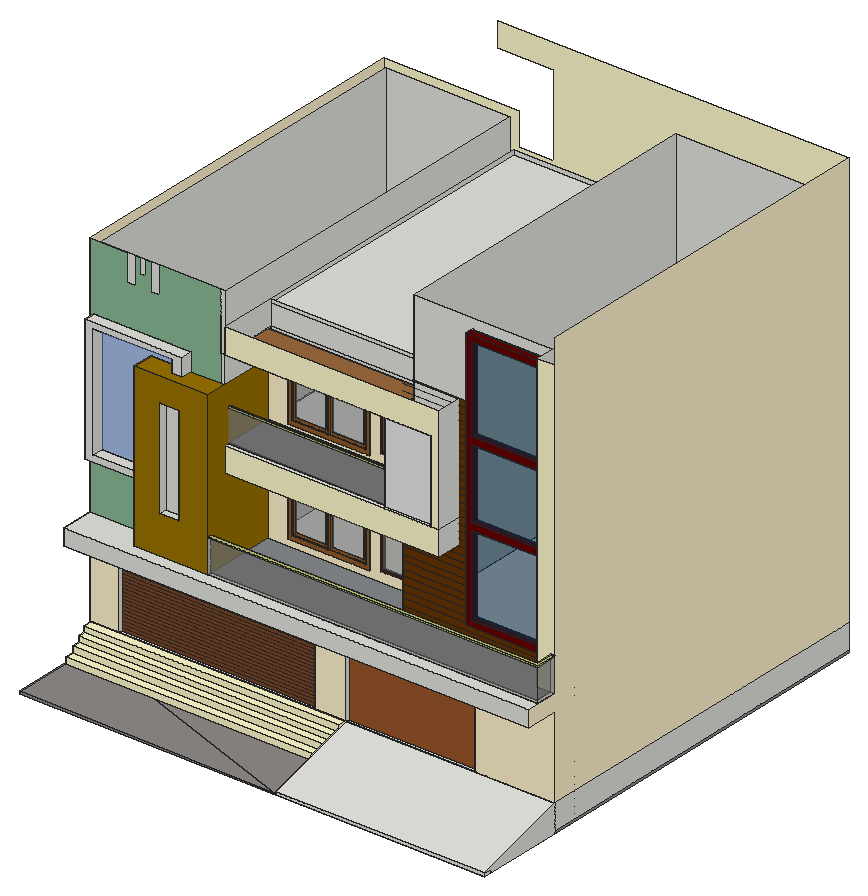
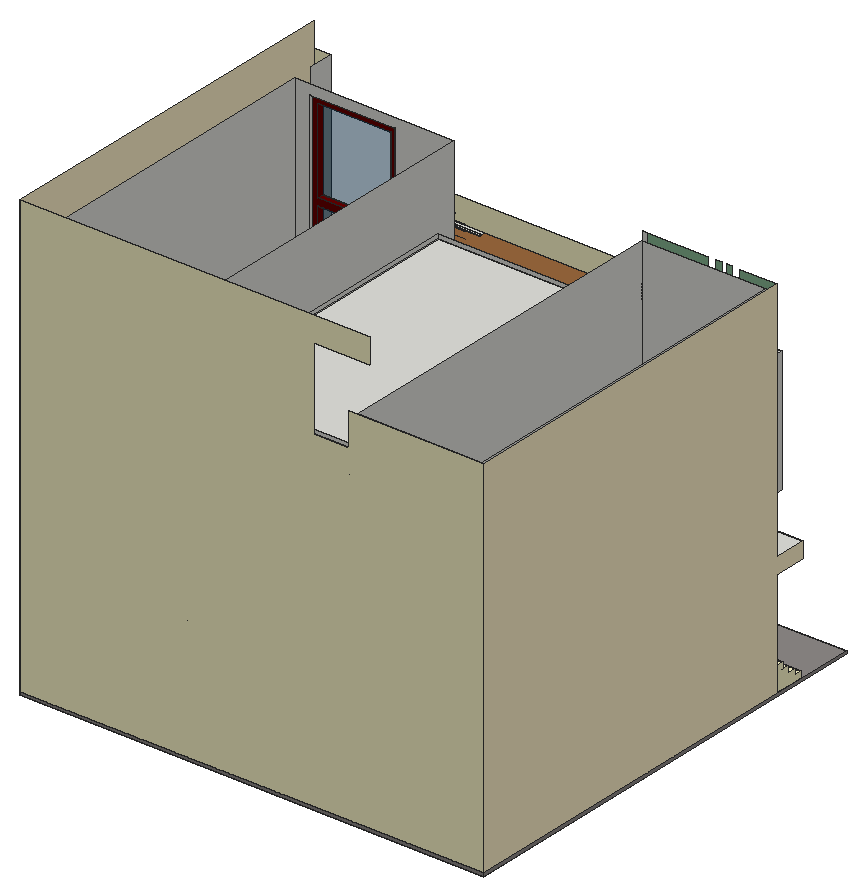
# SketchUp Ruby script. Lengths in inches.
U = 1.inch
M = Sketchup.active_model
def pt(a) = Geom::Point3d.new(a.map { |v| v * U })
def face(e, loops, mat)
  f = e.add_face(loops[0].map { |a| pt(a) })
  loops[1..].each { |l| e.add_face(l.map { |a| pt(a) }).erase! }
  f.material = f.back_material = mat if mat
  f
end
# faces: each face lists its corners as indices into pts; further lists are holes
def faces(e, pts, list, mat = nil) = list.each { |f| face(e, (f[0].is_a?(Array) ? f : [f]).map { |l| l.map { |i| pts[i] } }, mat) }
# xy, xz, yz: faces in a plane at the given z, y or x. An outline is a flat list of corners, or four numbers for a rectangle; further outlines are holes
def ring(l) = l.size == 4 ? [[l[0], l[1]], [l[2], l[1]], [l[2], l[3]], [l[0], l[3]]] : l.each_slice(2).to_a
def flat(e, list, mat, &to3) = list.each { |f| face(e, (f[0].is_a?(Array) ? f : [f]).map { |l| ring(l).map { |u, v| to3.(u, v) } }, mat) }
def xy(e, z, list, mat = nil) = flat(e, list, mat) { |x, y| [x, y, z] }
def xz(e, y, list, mat = nil) = flat(e, list, mat) { |x, z| [x, y, z] }
def yz(e, x, list, mat = nil) = flat(e, list, mat) { |y, z| [x, y, z] }
def lines(e, pts, list) = list.each { |a, b| e.add_line(pt(pts[a]), pt(pts[b])) }
# prism: a flat outline (further loops are holes) pulled along v
def prism(e, loops, v, mat = nil)
  f = face(e, loops, mat); d = Geom::Vector3d.new(v.map { |x| x * U })
  f.pushpull(f.normal.samedirection?(d) ? d.length : -d.length)
end
def box(e, o, s, mat = nil) = prism(e, [[o, [o[0] + s[0], o[1], o[2]], [o[0] + s[0], o[1] + s[1], o[2]], [o[0], o[1] + s[1], o[2]]]], [0, 0, s[2]], mat)
def at(x, y, z, deg = 0) = Geom::Transformation.translation(pt([x, y, z])) * Geom::Transformation.rotation(ORIGIN, Z_AXIS, deg.degrees)
def axes(o, x, y, z) = Geom::Transformation.new([*x, 0, *y, 0, *z, 0, *pt(o).to_a, 1])
def part(name) = M.definitions.add(name)
# library, detail: a bought-in or finely detailed component or shape, given as its bounding box
def library(name, o, s) = part(name).tap { |d| box(d.entities, o, s) }
def detail(e, o, s) = box(e.add_group.entities, o, s)
def put(e, d, t, mat = nil) = e.add_instance(d, t).tap { |i| i.material = mat if mat }
def group(e, t, mat = nil) = e.add_group.tap { |g| g.transformation = t; g.material = mat if mat }.entities
root = M.entities
M.materials.add("[0050_LemonChiffon]").color = [255, 250, 205]
M.materials.add("[0079_Teal]").color = [136, 184, 147]
M.materials.add("[Blacktop Old 01]").color = [132, 136, 139]
M.materials.add("[Color A08]").color = [102, 0, 0]
M.materials.add("[Color B08]").color = [102, 25, 0]
M.materials.add("[Color C08]").color = [102, 51, 0]
M.materials.add("[Color D01]").color = [255, 242, 204]
M.materials.add("[Color D07]").color = [153, 114, 0]
M.materials.add("[Herringbone 2x1]").color = [231, 231, 231]
M.materials.add("[Metal Corrugated Shiny]").color = [193, 193, 113]
M.materials.add("[Stone Marble]").color = [143, 138, 136]
M.materials.add("[Translucent Glass Blue]").color = [4, 53, 86]
M.materials["[Translucent Glass Blue]"].alpha = 0.5
M.materials.add("[Translucent Glass Blue]1").color = [100, 149, 237]
M.materials["[Translucent Glass Blue]1"].alpha = 0.5
M.materials.add("[Translucent Glass Gray]").color = [128, 128, 128]
M.materials["[Translucent Glass Gray]"].alpha = 0.5
M.materials.add("[Wood Cherry Original]").color = [152, 86, 42]
M.materials.add("[Wood Floor Parquet]").color = [145, 89, 39]
M.materials.add("[Wood Floor]").color = [155, 105, 61]
M.materials.add("[Wood Veneer 01]").color = [120, 70, 37]
c1 = part("Group\#2")
xy(c1.entities,0,[[0,0,217.625,6.75],[0,6.75,217.625,8.875]],"[Wood Floor Parquet]")
xy(c1.entities,10.46,[[10.46,0,106.8125,6.75],[108.8125,0,207.17,6.75],[10.46,6.75,106.8125,8.875],[108.8125,6.75,207.17,8.875]],"[Wood Floor Parquet]")
xy(c1.entities,17.65,[[17.65,6.75,99.62,8.875],[116.01,6.75,199.97,8.875]],"[Wood Floor Parquet]")
xy(c1.entities,173.85,[[17.65,6.75,99.62,8.875],[116.01,6.75,199.97,8.875]],"[Wood Floor Parquet]")
xy(c1.entities,181.04,[[10.46,0,106.8125,6.75],[108.8125,0,207.17,6.75],[10.46,6.75,106.8125,8.875],[108.8125,6.75,207.17,8.875]],"[Wood Floor Parquet]")
xy(c1.entities,191.5,[[0,0,217.625,6.75],[0,6.75,217.625,8.875]],"[Wood Floor Parquet]")
xz(c1.entities,0,[[[0,0,217.625,191.5],[108.8125,10.46,207.17,181.04],[10.46,10.46,106.8125,181.04]]],"[Wood Floor Parquet]")
xz(c1.entities,6.75,[[17.65,17.65,99.62,173.85],[116.01,17.65,199.97,173.85]],"[Translucent Glass Gray]")
xz(c1.entities,6.75,[[[0,0,217.625,191.5],[108.8125,10.46,207.17,181.04],[10.46,10.46,106.8125,181.04]],[[10.46,10.46,106.8125,181.04],[17.65,17.65,99.62,173.85]],[[108.8125,10.46,207.17,181.04],[116.01,17.65,199.97,173.85]]],"[Wood Floor Parquet]")
xz(c1.entities,8.875,[[[0,0,217.625,191.5],[108.8125,10.46,207.17,181.04],[10.46,10.46,106.8125,181.04]],[[10.46,10.46,106.8125,181.04],[17.65,17.65,99.62,173.85]],[[108.8125,10.46,207.17,181.04],[116.01,17.65,199.97,173.85]]],"[Wood Floor Parquet]")
yz(c1.entities,0,[[0,0,6.75,191.5],[6.75,0,8.875,191.5]],"[Wood Floor Parquet]")
yz(c1.entities,10.46,[[0,10.46,6.75,181.04],[6.75,10.46,8.875,181.04]],"[Wood Floor Parquet]")
yz(c1.entities,17.65,[[6.75,17.65,8.875,173.85]],"[Wood Floor Parquet]")
yz(c1.entities,99.62,[[6.75,17.65,8.875,173.85]],"[Wood Floor Parquet]")
yz(c1.entities,106.8125,[[0,10.46,6.75,181.04],[6.75,10.46,8.875,181.04]],"[Wood Floor Parquet]")
yz(c1.entities,108.8125,[[0,10.46,6.75,181.04],[6.75,10.46,8.875,181.04]],"[Wood Floor Parquet]")
yz(c1.entities,116.01,[[6.75,17.65,8.875,173.85]],"[Wood Floor Parquet]")
yz(c1.entities,199.97,[[6.75,17.65,8.875,173.85]],"[Wood Floor Parquet]")
yz(c1.entities,207.17,[[0,10.46,6.75,181.04],[6.75,10.46,8.875,181.04]],"[Wood Floor Parquet]")
yz(c1.entities,217.625,[[0,0,6.75,191.5],[6.75,0,8.875,191.5]],"[Wood Floor Parquet]")
c2 = part("Group\#3")
xy(c2.entities,0,[[0,0,43.875,1.8125],[0,1.8125,43.875,3.875]],"[Color B08]")
xy(c2.entities,1.78,[[1.78,0,42.09,1.8125],[1.78,1.8125,42.09,3.875]],"[Color B08]")
xy(c2.entities,69.21,[[1.78,0,42.09,1.8125],[1.78,1.8125,42.09,3.875]],"[Color B08]")
xy(c2.entities,70.99,[[0,0,43.875,1.8125],[0,1.8125,43.875,3.875]],"[Color B08]")
xz(c2.entities,0,[[[0,0,43.875,70.99],[1.78,1.78,42.09,69.21]]],"[Color B08]")
xz(c2.entities,1.8125,[[[0,0,43.875,70.99],[1.78,1.78,42.09,69.21]]],"[Color B08]")
xz(c2.entities,1.8125,[[1.78,1.78,42.09,69.21]],"[Translucent Glass Gray]")
xz(c2.entities,3.875,[[[0,0,43.875,70.99],[1.78,1.78,42.09,69.21]]],"[Color B08]")
yz(c2.entities,0,[[0,0,1.8125,70.99],[1.8125,0,3.875,70.99]],"[Color B08]")
yz(c2.entities,1.78,[[0,1.78,1.8125,69.21],[1.8125,1.78,3.875,69.21]],"[Color B08]")
yz(c2.entities,42.09,[[0,1.78,1.8125,69.21],[1.8125,1.78,3.875,69.21]],"[Color B08]")
yz(c2.entities,43.875,[[0,0,1.8125,70.99],[1.8125,0,3.875,70.99]],"[Color B08]")
xy(root,0,[[0,0,0,668.625,682.125,668.625,682.125,128.625,375.57,128.625,375.57,0],[375.57,0,682.125,11.625],[375.57,11.625,682.125,128.625]])
xy(root,4.03,[[375.57,0,682.125,11.625]])
xy(root,40,[[42.48,128.625,329.85,133.375],[375.57,128.625,565.32,133.375],[9,137.625,591,659.625]])
xy(root,140.3125,[[42.48,128.625,329.85,133.375],[375.57,128.625,565.32,133.375]])
xy(root,154,[[9,137.625,591,659.625]])
xy(root,160,[[0,80.8125,682.125,128.625],[9,137.625,591,659.625]])
xy(root,184,[[0,80.8125,682.125,80.8125,682.125,97.8125,89.4375,97.8125,89.4375,128.625,0,128.625],[191.5625,97.8125,197.5625,137.625],[197.5625,97.8125,197.5625,103.64,677.375,103.64,677.375,128.625,682.125,128.625,682.125,97.8125],[9,137.625,191.5625,659.625],[436.125,177.0625,671.25,659.625],
  [197.5625,214.0625,429.93,659.625],[429.93,214.0625,436.125,659.625]])
xy(root,184,[[197.5625,103.64,677.375,103.64,677.375,128.625,656.59,128.625,656.59,165,430.125,165,430.125,208.0625,197.5625,208.0625]],"[Blacktop Old 01]")
xy(root,193.03,[[226.36,208.0625,346.92,214.0625]])
xy(root,197.79,[[363.4,208.0625,417.52,214.0625]])
xy(root,202.44,[[523.3,165,648.11,177.0625]])
xy(root,232,[[197.5625,97.8125,197.5625,103.64,677.375,103.64,677.375,128.625,682.125,128.625,682.125,97.8125]],"[Metal Corrugated Shiny]")
xy(root,234,[[197.5625,97.8125,682.125,97.8125,682.125,128.625,677.375,128.625,677.375,103.64,197.5625,103.64]],"[Metal Corrugated Shiny]")
xy(root,239.63,[[127.625,97.8125,154.9375,108.5625]])
xy(root,262.85,[[5.75,111.9375,89.4375,128.625]])
xy(root,272.03,[[17.76,111.9375,89.4375,128.625]])
xy(root,293.6,[[363.4,208.0625,417.52,214.0625]])
xy(root,297.78,[[226.36,208.0625,346.92,214.0625]])
xy(root,304,[[197.5625,128.625,197.5625,208.0625,430.125,208.0625,430.125,165,512.0625,165,512.0625,128.625]],"[Wood Floor]")
xy(root,340,[[197.5625,128.625,500.51,128.625,500.51,132.9375,430.125,132.9375,430.125,133.875,197.5625,133.875],[197.5625,133.875,430.125,135.875],[197.5625,214.0625,429.93,659.625]])
xy(root,340,[[197.5625,135.875,430.125,135.875,430.125,137.55,500.51,137.55,500.51,165,430.125,165,430.125,208.0625,197.5625,208.0625]],"[Blacktop Old 01]")
xy(root,344.6,[[226.36,208.0625,346.92,214.0625]])
xy(root,352.47,[[363.4,208.0625,417.52,214.0625]])
xy(root,385.19,[[127.625,97.8125,154.9375,108.5625]])
xy(root,388,[[197.5625,133.875,430.125,135.875]],"[Metal Corrugated Shiny]")
xy(root,390.0625,[[197.5625,133.875,430.125,135.875]],"[Metal Corrugated Shiny]")
xy(root,420.1,[[132.83,111.9375,148.5625,128.625]])
xy(root,420.1,[[89.4375,97.8125,197.5625,97.8125,197.5625,128.625,148.5625,128.625,148.5625,111.9375,132.83,111.9375,132.83,128.625,89.4375,128.625]],"[Color D07]")
xy(root,438.47,[[17.76,111.9375,132.83,128.625]])
xy(root,446.32,[[5.75,111.9375,148.5625,128.625]])
xy(root,448.29,[[363.4,208.0625,417.52,214.0625]])
xy(root,449.35,[[226.36,208.0625,346.92,214.0625]])
xy(root,460,[[430.125,128.625,500.51,132.9375],[430.125,132.9375,500.51,137.55]])
xy(root,460,[[197.5625,128.625,197.5625,208.0625,430.125,208.0625,430.125,165,500.51,165,500.51,137.55,430.125,137.55,430.125,128.625]],"[Wood Floor]")
xy(root,490,[[197.5625,214.0625,429.93,659.625]])
xz(root,0,[[375.57,0,682.125,4.03]])
xz(root,0,[[0,0,375.57,0,375.57,0.4,0,4]],"[Stone Marble]")
xz(root,11.625,[[375.57,0,682.125,4.03]])
xz(root,80.8125,[[0,160,682.125,184]])
xz(root,97.8125,[[[89.4375,184,197.5625,420.1],[127.625,239.63,154.9375,385.19]]],"[Color D07]")
xz(root,97.8125,[[197.5625,232,682.125,234]],"[Metal Corrugated Shiny]")
xz(root,97.8125,[[197.5625,184,682.125,232]],"[Translucent Glass Gray]")
xz(root,103.64,[[197.5625,232,677.375,234]],"[Metal Corrugated Shiny]")
xz(root,103.64,[[197.5625,184,677.375,232]],"[Translucent Glass Gray]")
xz(root,108.5625,[[127.625,239.63,154.9375,385.19]])
xz(root,111.9375,[[5.75,262.85,89.4375,262.85,89.4375,272.03,17.76,272.03,17.76,438.47,132.83,438.47,132.83,420.1,148.5625,420.1,148.5625,446.32,5.75,446.32]])
xz(root,128.625,[[375.57,0,682.125,40],[0,4,375.57,40],[677.375,184,682.125,232],[5.75,262.85,5.75,446.32,148.5625,446.32,148.5625,420.1,132.83,420.1,132.83,438.47,17.76,438.47,17.76,272.03,89.4375,272.03,89.4375,262.85],[191.5625,420.1,197.5625,460],
  [191.5625,460,197.5625,544]])
xz(root,128.625,[[656.59,184,677.375,184,677.375,234,682.125,234,682.125,616,656.59,616],[197.5625,304,512.0625,340],[500.51,340,512.0625,340,512.0625,496,197.5625,496,197.5625,460,500.51,460]],"[0050_LemonChiffon]")
xz(root,128.625,[[0,184,89.4375,184,89.4375,262.85,5.75,262.85,5.75,446.32,148.5625,446.32,148.5625,420.1,191.5625,420.1,191.5625,544,101.91,544,101.91,504.9375,89.6,504.9375,89.6,544,81.29,544,81.29,522.8125,73.73,522.8125,73.73,544,66.79,544,66.79,504.9375,54.48,504.9375,54.48,544,0,544]],"[0079_Teal]")
xz(root,128.625,[[0,40,42.48,40,42.48,140.3125,329.85,140.3125,329.85,40,375.57,40,375.57,140.3125,565.32,140.3125,565.32,40,682.125,40,682.125,160,0,160]],"[Color D01]")
xz(root,128.625,[[677.375,232,682.125,234]],"[Metal Corrugated Shiny]")
xz(root,128.625,[[17.76,272.03,89.4375,272.03,89.4375,420.1,132.83,420.1,132.83,438.47,17.76,438.47]],"[Translucent Glass Blue]1")
xz(root,132.9375,[[430.125,340,500.51,460]],"[Herringbone 2x1]")
xz(root,133.375,[[375.57,40,565.32,140.3125]],"[Wood Cherry Original]")
xz(root,133.375,[[42.48,40,329.85,134.6875],[42.48,134.6875,329.85,140.3125]],"[Wood Veneer 01]")
xz(root,133.875,[[197.5625,388,430.125,390.0625]],"[Metal Corrugated Shiny]")
xz(root,133.875,[[197.5625,340,430.125,388]],"[Translucent Glass Gray]")
xz(root,135.875,[[197.5625,388,430.125,390.0625]],"[Metal Corrugated Shiny]")
xz(root,135.875,[[197.5625,340,430.125,388]],"[Translucent Glass Gray]")
xz(root,137.55,[[430.125,340,500.51,460]])
xz(root,137.625,[[9,40,591,154],[9,154,591,160],[9,184,191.5625,538]])
xz(root,165,[[430.125,184,656.59,185.6],[430.125,185.6,656.59,195.35],[430.125,195.35,656.59,195.35,656.59,205.1,648.11,205.1,648.11,202.44,523.3,202.44,523.3,205.1,430.125,205.1],[430.125,205.1,523.3,214.85],[648.11,205.1,656.59,214.85],
  [430.125,214.85,523.3,224.6],[648.11,214.85,656.59,224.6],[430.125,224.6,523.3,234.35],[648.11,224.6,656.59,234.35],[430.125,234.35,523.3,244.1],
  [648.11,234.35,656.59,244.1],[430.125,244.1,523.3,253.85],[648.11,244.1,656.59,253.85],[430.125,253.85,523.3,263.6],[648.11,253.85,656.59,263.6],
  [430.125,263.6,523.3,273.35],[648.11,263.6,656.59,273.35],[430.125,273.35,523.3,283.1],[648.11,273.35,656.59,283.1],[430.125,283.1,523.3,292.85],
  [648.11,283.1,656.59,292.85],[430.125,292.85,523.3,302.6],[648.11,292.85,656.59,302.6],[430.125,302.6,523.3,302.6,523.3,312.35,512.0625,312.35,512.0625,304,430.125,304],[648.11,302.6,656.59,312.35],
  [512.0625,312.35,523.3,322.1],[648.11,312.35,656.59,322.1],[512.0625,322.1,523.3,331.85],[648.11,322.1,656.59,331.85],[512.0625,331.85,523.3,341.6],
  [648.11,331.85,656.59,341.6],[430.125,340,500.51,341.6],[430.125,341.6,500.51,351.35],[512.0625,341.6,523.3,351.35],[648.11,341.6,656.59,351.35],
  [430.125,351.35,500.51,361.1],[512.0625,351.35,523.3,361.1],[648.11,351.35,656.59,361.1],[430.125,361.1,500.51,370.85],[512.0625,361.1,523.3,370.85],
  [648.11,361.1,656.59,370.85],[430.125,370.85,500.51,380.6],[512.0625,370.85,523.3,380.6],[648.11,370.85,656.59,380.6],[430.125,380.6,500.51,390.35],
  [512.0625,380.6,523.3,390.35],[648.11,380.6,656.59,390.35],[430.125,390.35,500.51,400.1],[512.0625,390.35,523.3,400.1],[648.11,390.35,656.59,400.1],
  [430.125,400.1,500.51,409.85],[512.0625,400.1,523.3,409.85],[648.11,400.1,656.59,409.85],[430.125,409.85,500.51,419.6],[512.0625,409.85,523.3,419.6],
  [648.11,409.85,656.59,419.6],[430.125,419.6,500.51,429.35],[512.0625,419.6,523.3,429.35],[648.11,419.6,656.59,429.35],[430.125,429.35,500.51,439.1],
  [512.0625,429.35,523.3,439.1],[648.11,429.35,656.59,439.1],[430.125,439.1,500.51,448.85],[512.0625,439.1,523.3,448.85],[648.11,439.1,656.59,448.85],
  [430.125,448.85,500.51,458.6],[512.0625,448.85,523.3,458.6],[648.11,448.85,656.59,458.6],[430.125,458.6,500.51,460],[512.0625,458.6,523.3,468.35],
  [648.11,458.6,656.59,468.35],[512.0625,468.35,523.3,478.1],[648.11,468.35,656.59,478.1],[512.0625,478.1,523.3,487.85],[648.11,478.1,656.59,487.85],
  [512.0625,487.85,523.3,487.85,523.3,497.6,444.53,497.6,444.53,496,512.0625,496],[648.11,487.85,656.59,497.6]],"[Color C08]")
xz(root,177.0625,[[[436.125,184,671.25,601.3125],[523.3,202.44,648.11,587.25]]])
xz(root,208.0625,[[[197.5625,184,430.125,304],[226.36,193.03,346.92,297.78],[363.4,197.79,417.52,293.6]],[[197.5625,340,430.125,460],[226.36,344.6,346.92,449.35],[363.4,352.47,417.52,448.29]]],"[Color D01]")
xz(root,214.0625,[[[197.5625,184,429.93,304],[226.36,193.03,346.92,297.78],[363.4,197.79,417.52,293.6]],[197.5625,304,429.93,340],[[197.5625,340,429.93,460],[226.36,344.6,346.92,449.35],[363.4,352.47,417.52,448.29]],[197.5625,460,429.93,490],[197.5625,490,429.93,496]])
xz(root,659.625,[[9,40,591,154],[9,154,67.5625,160],[67.5625,154,591,160],[9,160,67.5625,184],[9,184,191.5625,538],
  [197.5625,184,429.93,304],[429.93,184,436.125,304],[436.125,184,671.25,601.3125],[197.5625,304,429.93,340],[429.93,304,436.125,340],
  [197.5625,340,429.93,460],[429.93,340,436.125,460],[429.93,460,436.125,496],[197.5625,490,429.93,496]])
xz(root,668.625,[[0,4,0,544,197.5625,544,197.5625,496,249,496,249,616,167.125,616,167.125,652,682.125,652,682.125,4]],"[0050_LemonChiffon]")
xz(root,668.625,[[0,0,682.125,4]],"[Stone Marble]")
yz(root,0,[[128.625,4,128.625,160,80.8125,160,80.8125,184,128.625,184,128.625,544,668.625,544,668.625,4]],"[Color D01]")
yz(root,0,[[0,0,668.625,4]],"[Stone Marble]")
yz(root,5.75,[[111.9375,262.85,128.625,446.32]])
yz(root,9,[[137.625,40,659.625,154],[137.625,154,659.625,160],[137.625,160,659.625,184],[137.625,184,659.625,538]])
yz(root,17.76,[[111.9375,272.03,128.625,438.47]])
yz(root,42.48,[[128.625,40,133.375,140.3125]])
yz(root,89.4375,[[111.9375,262.85,128.625,272.03]])
yz(root,89.4375,[[97.8125,184,97.8125,420.1,128.625,420.1,128.625,272.03,111.9375,272.03,111.9375,262.85,128.625,262.85,128.625,184]],"[Color D07]")
yz(root,127.625,[[97.8125,239.63,108.5625,385.19]])
yz(root,132.83,[[111.9375,420.1,128.625,438.47]])
yz(root,148.5625,[[111.9375,420.1,128.625,446.32]])
yz(root,154.9375,[[97.8125,239.63,108.5625,385.19]])
yz(root,191.5625,[[137.625,184,659.625,538],[128.625,460,137.625,508]])
yz(root,197.5625,[[97.8125,184,103.64,232],[214.0625,184,659.625,304],[214.0625,304,659.625,340],[133.875,340,135.875,388],[214.0625,340,659.625,460],
  [128.625,420.1,208.0625,460],[128.625,460,214.0625,496],[214.0625,490,659.625,496]])
yz(root,197.5625,[[103.64,184,208.0625,184,208.0625,304,128.625,304,128.625,340,133.875,340,133.875,390.0625,135.875,390.0625,135.875,340,208.0625,340,208.0625,420.1,97.8125,420.1,97.8125,234,103.64,234]],"[Color D07]")
yz(root,197.5625,[[97.8125,232,103.64,234],[133.875,388,135.875,390.0625]],"[Metal Corrugated Shiny]")
yz(root,226.36,[[208.0625,193.03,214.0625,297.78],[208.0625,344.6,214.0625,449.35]])
yz(root,329.85,[[128.625,40,133.375,140.3125]])
yz(root,346.92,[[208.0625,193.03,214.0625,297.78],[208.0625,344.6,214.0625,449.35]])
yz(root,363.4,[[208.0625,197.79,214.0625,293.6],[208.0625,352.47,214.0625,448.29]])
yz(root,375.57,[[0,0,11.625,0.4],[11.625,0,128.625,0,128.625,4,11.625,0.73],[0,0.4,0,4.03,11.625,4.03,11.625,0.73],[0,0.4,11.625,0.4,11.625,0.73],[11.625,0.73,11.625,4.03,0,4.03,128.625,40,128.625,4],
  [128.625,40,133.375,140.3125]])
yz(root,417.52,[[208.0625,197.79,214.0625,293.6],[208.0625,352.47,214.0625,448.29]])
yz(root,429.93,[[214.0625,184,659.625,340],[214.0625,340,659.625,490],[214.0625,490,659.625,496]])
yz(root,430.125,[[132.9375,340,132.9375,460,137.55,460,137.55,340,135.875,340,135.875,390.0625,133.875,390.0625,133.875,340],[133.875,340,135.875,388]])
yz(root,430.125,[[165,184,208.0625,304],[165,340,208.0625,460]],"[Color C08]")
yz(root,430.125,[[133.875,388,135.875,390.0625]],"[Metal Corrugated Shiny]")
yz(root,436.125,[[177.0625,184,659.625,601.3125]])
yz(root,500.51,[[128.625,340,132.9375,460],[132.9375,340,137.55,460],[137.55,340,165,460]])
yz(root,512.0625,[[128.625,304,165,340],[128.625,340,165,496]])
yz(root,523.3,[[165,202.44,177.0625,587.25]])
yz(root,565.32,[[128.625,40,133.375,140.3125]])
yz(root,591,[[137.625,40,659.625,154],[137.625,154,659.625,160]])
yz(root,648.11,[[165,202.44,177.0625,587.25]])
yz(root,656.59,[[128.625,184,165,616]])
yz(root,671.25,[[177.0625,184,659.625,601.3125]])
yz(root,677.375,[[103.64,232,128.625,234]],"[Metal Corrugated Shiny]")
yz(root,677.375,[[103.64,184,128.625,232]],"[Translucent Glass Gray]")
yz(root,682.125,[[0,0,11.625,4.03],[11.625,0,128.625,0,128.625,40,0,4.03,11.625,4.03],[128.625,4,668.625,40]])
yz(root,682.125,[[128.625,40,668.625,40,668.625,652,128.625,652,128.625,184,80.8125,184,80.8125,160,128.625,160]],"[Color D01]")
yz(root,682.125,[[97.8125,232,128.625,234]],"[Metal Corrugated Shiny]")
yz(root,682.125,[[128.625,0,668.625,4]],"[Stone Marble]")
yz(root,682.125,[[97.8125,184,128.625,232]],"[Translucent Glass Gray]")
p = [[0,0,4],[375.57,0,0.4],[0,128.625,4],[375.57,128.625,4],[375.57,11.625,0.73],[375.57,0,4.03],
  [682.125,0,4.03],[682.125,128.625,40],[565.32,128.625,40],[375.57,128.625,40],[591,659.625,160],[591,659.625,184],
  [191.5625,137.625,304],[191.5625,128.625,304],[191.5625,137.625,340],[191.5625,128.625,340],[436.125,214.0625,340],[429.93,214.0625,340],
  [436.125,214.0625,460],[429.93,214.0625,460],[197.5625,668.625,460],[197.5625,659.625,460],[436.125,659.625,184],[436.125,668.625,184],
  [430.125,165,487.85],[512.0625,165,487.85],[430.125,165,478.1],[512.0625,165,478.1],[430.125,165,468.35],[512.0625,165,468.35],
  [430.125,165,331.85],[512.0625,165,331.85],[430.125,165,322.1],[512.0625,165,322.1],[430.125,165,312.35],[512.0625,165,312.35],
  [656.59,165,175.85],[682.125,165,175.85],[430.125,165,175.85],[512.0625,165,175.85],[656.59,165,166.1],[682.125,165,166.1],
  [430.125,165,166.1],[512.0625,165,166.1],[430.125,165,156.35],[512.0625,165,156.35],[430.125,165,146.6],[512.0625,165,146.6],
  [430.125,165,136.85],[512.0625,165,136.85],[430.125,165,127.1],[512.0625,165,127.1],[430.125,165,117.35],[512.0625,165,117.35],
  [430.125,165,107.6],[512.0625,165,107.6],[430.125,165,97.85],[512.0625,165,97.85],[430.125,165,88.1],[512.0625,165,88.1],
  [656.59,165,78.35],[682.125,165,78.35],[430.125,165,78.35],[512.0625,165,78.35],[430.125,165,68.6],[512.0625,165,68.6],
  [656.59,165,58.85],[682.125,165,58.85],[430.125,165,58.85],[512.0625,165,58.85],[656.59,165,49.1],[682.125,165,49.1],
  [430.125,165,49.1],[512.0625,165,49.1],[656.59,165,39.35],[682.125,165,39.35],[430.125,165,39.35],[512.0625,165,39.35],
  [656.59,165,29.6],[682.125,165,29.6],[430.125,165,29.6],[512.0625,165,29.6],[656.59,165,19.85],[682.125,165,19.85],
  [430.125,165,19.85],[512.0625,165,19.85],[656.59,165,10.1],[682.125,165,10.1],[430.125,165,10.1],[512.0625,165,10.1],
  [42.72,133.375,129.94],[329.85,133.375,129.94],[330.1,133.375,129.94],[42.97,133.375,125.2],[329.85,133.375,125.2],[330.34,133.375,125.2],
  [43.21,133.375,120.46],[329.85,133.375,120.46],[330.59,133.375,120.46],[43.46,133.375,115.71],[329.85,133.375,115.71],[330.84,133.375,115.71],
  [43.71,133.375,110.97],[329.85,133.375,110.97],[331.08,133.375,110.97],[43.95,133.375,106.23],[329.85,133.375,106.23],[331.33,133.375,106.23],
  [44.2,133.375,101.48],[329.85,133.375,101.48],[331.57,133.375,101.48],[44.44,133.375,96.74],[329.85,133.375,96.74],[331.82,133.375,96.74],
  [44.69,133.375,91.99],[329.85,133.375,91.99],[332.07,133.375,91.99],[44.9375,133.375,87.25],[329.85,133.375,87.25],[332.3125,133.375,87.25],
  [45.18,133.375,82.51],[329.85,133.375,82.51],[332.56,133.375,82.51],[45.43,133.375,77.76],[329.85,133.375,77.76],[332.8,133.375,77.76],
  [45.68,133.375,73.02],[329.85,133.375,73.02],[333.05,133.375,73.02],[45.92,133.375,68.28],[329.85,133.375,68.28],[333.3,133.375,68.28],
  [46.17,133.375,63.53],[329.85,133.375,63.53],[333.54,133.375,63.53],[46.41,133.375,58.79],[329.85,133.375,58.79],[333.79,133.375,58.79],
  [46.66,133.375,54.05],[329.85,133.375,54.05],[334.03,133.375,54.05],[46.91,133.375,49.3],[329.85,133.375,49.3],[334.28,133.375,49.3],
  [47.15,133.375,44.56],[329.85,133.375,44.56],[334.53,133.375,44.56],[47.4,133.375,39.82],[334.77,133.375,39.82],[47.64,133.375,35.07],
  [335.02,133.375,35.07],[47.89,133.375,30.33],[335.27,133.375,30.33],[48.14,133.375,25.58],[335.51,133.375,25.58],[48.38,133.375,20.84],
  [335.76,133.375,20.84],[48.63,133.375,16.1],[336,133.375,16.1],[48.875,133.375,11.35],[336.25,133.375,11.35],[49.12,133.375,6.61],
  [336.5,133.375,6.61],[49.37,133.375,1.87],[336.74,133.375,1.87]]
faces(root,p,[[0,1,2],[3,2,1,4]],"[Stone Marble]")
faces(root,p,[[5,6,7,8,9]])
lines(root,p,[[10,11],[12,13],[14,15],[16,17],[18,19],[20,21],[22,23],[24,25],[26,27],[28,29],[30,31],[32,33],
  [34,35],[36,37],[38,39],[39,36],[40,41],[42,43],[43,40],[44,45],[46,47],[48,49],[50,51],[52,53],
  [54,55],[56,57],[58,59],[60,61],[62,63],[64,65],[66,67],[68,69],[70,71],[72,73],[74,75],[76,77],
  [78,79],[80,81],[81,78],[82,83],[84,85],[85,82],[86,87],[88,89],[89,86],[90,91],[91,92],[93,94],
  [94,95],[96,97],[97,98],[99,100],[100,101],[102,103],[103,104],[105,106],[106,107],[108,109],[109,110],[111,112],
  [112,113],[114,115],[115,116],[117,118],[118,119],[120,121],[121,122],[123,124],[124,125],[126,127],[127,128],[129,130],
  [130,131],[132,133],[133,134],[135,136],[136,137],[138,139],[139,140],[141,142],[142,143],[144,145],[145,146],[147,148],
  [149,150],[151,152],[153,154],[155,156],[157,158],[159,160],[161,162],[163,164]])
g1 = group(root,at(1.01,82.86,4),"[0050_LemonChiffon]")
prism(g1,[[[0,0,8.96],[0,12,8.96],[0,12,17.92],[0,24,17.92],[0,24,26.88],[0,33.76,26.88],[0,33.76,35.84],[0,45.76,35.84],[0,45.76,26.88],[0,45.76,0],[0,12,0],[0,0,0]]],[374.57,0,0])
p = [[0,33.76,26.88],[0,36,26.88],[374.57,36,26.88]]
lines(g1,p,[[0,1],[1,2]])
put(root,c1,axes([226.36,208.0625,193.03],[0.55399,0,0],[0,0.345,0],[0,0,0.547]))
put(root,c2,axes([363.4,208.0625,197.79],[1.23362,0,0],[0,1,0],[0,0,1.34964]))
g2 = group(root,at(523.3,165,202.44))
xy(g2,0,[[0,0,124.8125,9.1875]],"[Color A08]")
xy(g2,9.11,[[8.31,0,116.51,9.1875]],"[Color A08]")
xy(g2,127.4375,[[8.31,0,116.51,9.1875]],"[Color A08]")
xy(g2,137.67,[[8.31,0,116.51,9.1875]],"[Color A08]")
xy(g2,240.45,[[8.31,0,116.51,9.1875]],"[Color A08]")
xy(g2,250.68,[[8.31,0,116.51,9.1875]],"[Color A08]")
xy(g2,375.7,[[8.31,0,116.51,9.1875]],"[Color A08]")
xy(g2,384.8125,[[0,0,124.8125,9.1875]],"[Color A08]")
xz(g2,0,[[[0,0,124.8125,384.8125],[8.31,250.68,116.51,375.7],[8.31,9.11,116.51,127.4375],[8.31,137.67,116.51,240.45]]],"[Color A08]")
xz(g2,0,[[8.31,9.11,116.51,127.4375],[8.31,137.67,116.51,240.45],[8.31,250.68,116.51,375.7]],"[Translucent Glass Blue]")
xz(g2,9.1875,[[[0,0,124.8125,384.8125],[8.31,250.68,116.51,375.7],[8.31,9.11,116.51,127.4375],[8.31,137.67,116.51,240.45]]],"[Color A08]")
yz(g2,0,[[0,0,9.1875,384.8125]],"[Color A08]")
yz(g2,8.31,[[0,9.11,9.1875,127.4375],[0,137.67,9.1875,240.45],[0,250.68,9.1875,375.7]],"[Color A08]")
yz(g2,116.51,[[0,9.11,9.1875,127.4375],[0,137.67,9.1875,240.45],[0,250.68,9.1875,375.7]],"[Color A08]")
yz(g2,124.8125,[[0,0,9.1875,384.8125]],"[Color A08]")
put(root,c1,axes([226.36,208.0625,344.6],[0.55399,0,0],[0,0.345,0],[0,0,0.547]))
put(root,c2,axes([363.4,208.0625,352.47],[1.23362,0,0],[0,1,0],[0,0,1.34964]))
